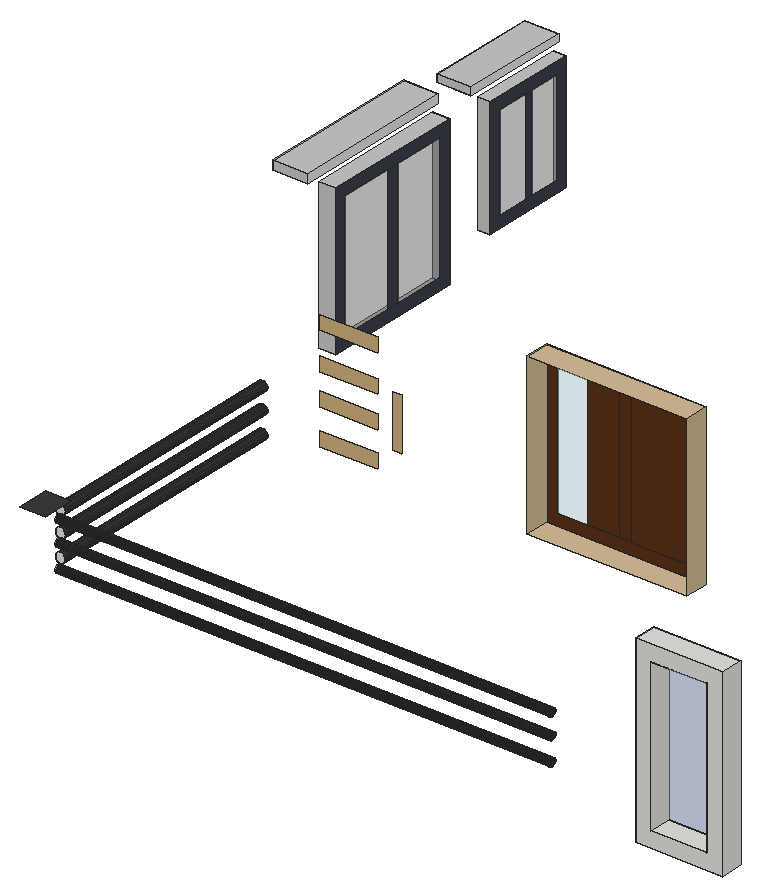
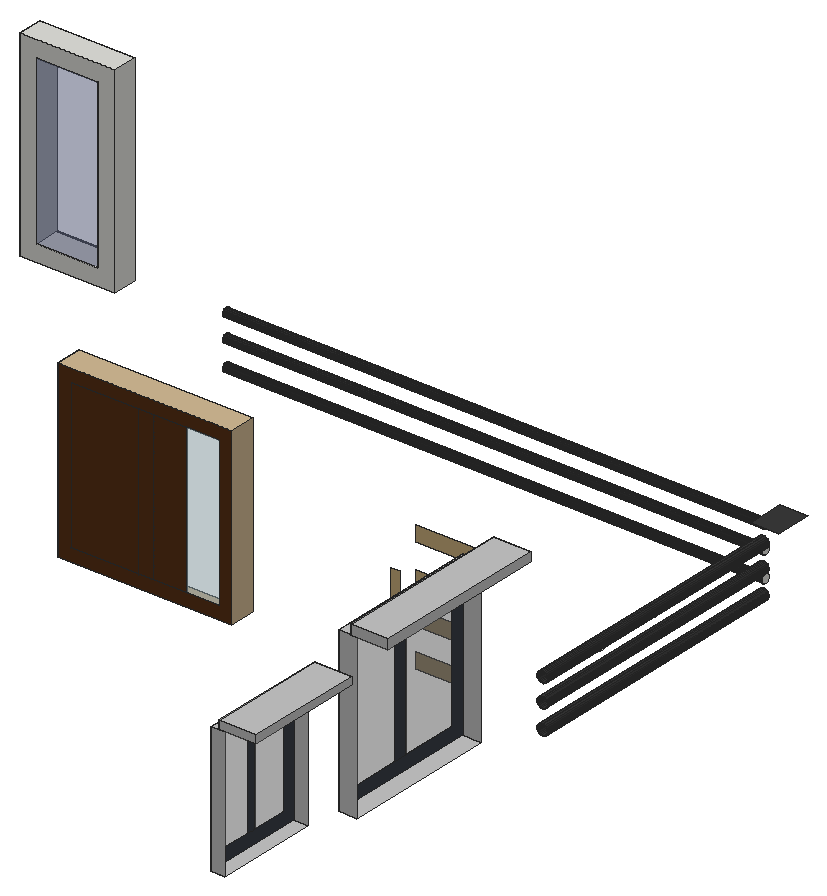
# SketchUp Ruby script. Lengths in inches.
U = 1.inch
M = Sketchup.active_model
def pt(a) = Geom::Point3d.new(a.map { |v| v * U })
def face(e, loops, mat)
  f = e.add_face(loops[0].map { |a| pt(a) })
  loops[1..].each { |l| e.add_face(l.map { |a| pt(a) }).erase! }
  f.material = f.back_material = mat if mat
  f
end
# faces: each face lists its corners as indices into pts; further lists are holes
def faces(e, pts, list, mat = nil) = list.each { |f| face(e, (f[0].is_a?(Array) ? f : [f]).map { |l| l.map { |i| pts[i] } }, mat) }
# xy, xz, yz: faces in a plane at the given z, y or x. An outline is a flat list of corners, or four numbers for a rectangle; further outlines are holes
def ring(l) = l.size == 4 ? [[l[0], l[1]], [l[2], l[1]], [l[2], l[3]], [l[0], l[3]]] : l.each_slice(2).to_a
def flat(e, list, mat, &to3) = list.each { |f| face(e, (f[0].is_a?(Array) ? f : [f]).map { |l| ring(l).map { |u, v| to3.(u, v) } }, mat) }
def xy(e, z, list, mat = nil) = flat(e, list, mat) { |x, y| [x, y, z] }
def xz(e, y, list, mat = nil) = flat(e, list, mat) { |x, z| [x, y, z] }
def yz(e, x, list, mat = nil) = flat(e, list, mat) { |y, z| [x, y, z] }
def lines(e, pts, list) = list.each { |a, b| e.add_line(pt(pts[a]), pt(pts[b])) }
# prism: a flat outline (further loops are holes) pulled along v
def prism(e, loops, v, mat = nil)
  f = face(e, loops, mat); d = Geom::Vector3d.new(v.map { |x| x * U })
  f.pushpull(f.normal.samedirection?(d) ? d.length : -d.length)
end
def box(e, o, s, mat = nil) = prism(e, [[o, [o[0] + s[0], o[1], o[2]], [o[0] + s[0], o[1] + s[1], o[2]], [o[0], o[1] + s[1], o[2]]]], [0, 0, s[2]], mat)
def at(x, y, z, deg = 0) = Geom::Transformation.translation(pt([x, y, z])) * Geom::Transformation.rotation(ORIGIN, Z_AXIS, deg.degrees)
def axes(o, x, y, z) = Geom::Transformation.new([*x, 0, *y, 0, *z, 0, *pt(o).to_a, 1])
def part(name) = M.definitions.add(name)
# library, detail: a bought-in or finely detailed component or shape, given as its bounding box
def library(name, o, s) = part(name).tap { |d| box(d.entities, o, s) }
def detail(e, o, s) = box(e.add_group.entities, o, s)
def put(e, d, t, mat = nil) = e.add_instance(d, t).tap { |i| i.material = mat if mat }
def group(e, t, mat = nil) = e.add_group.tap { |g| g.transformation = t; g.material = mat if mat }.entities
root = M.entities
M.materials.add("[Color M02]").color = [198, 198, 198]
M.materials.add("[Color M07]").color = [58, 58, 58]
M.materials.add("[Formica Beige]").color = [211, 187, 149]
M.materials.add("[Formica Laminate Dark]").color = [59, 63, 71]
M.materials.add("[Translucent Glass Gray]").color = [128, 128, 128]
M.materials["[Translucent Glass Gray]"].alpha = 0.5
M.materials.add("[Translucent Glass Safety]").color = [204, 235, 244]
M.materials["[Translucent Glass Safety]"].alpha = 0.5
M.materials.add("[Translucent Glass Sky Reflection]").color = [126, 138, 183]
M.materials["[Translucent Glass Sky Reflection]"].alpha = 0.52
M.materials.add("[Wood Cherry Original]").color = [89, 50, 24]
M.materials.add("[Wood Floor Light]").color = [204, 176, 127]
xy(root,525.6875,[[382.62,382.59,423.93,393.34]])
xy(root,526.85,[[206.59,538.2,282.28,549.76]],"[Formica Beige]")
xy(root,533.08,[[390.01,382.59,416.53,393.34]])
xy(root,541.0625,[[73.92,580.21,81.98,647.71]],"[Color M02]")
xy(root,544.4375,[[79.76,506.9375,80.23,507,80.66,507.18,81.04,507.47,81.33,507.84,81.51,508.28,81.57,508.75,81.51,509.22,81.33,509.66,81.04,510.03,80.66,510.32,80.23,510.5,79.76,510.5625,79.29,510.5,78.85,510.32,78.48,510.03,78.1875,509.66,78.01,509.22,77.95,508.75,78.01,508.28,78.1875,507.84,78.48,507.47,78.85,507.18,79.29,507]])
xy(root,544.75,[[79.76,478.5,80.23,478.5625,80.66,478.74,81.04,479.03,81.33,479.41,81.51,479.84,81.57,480.3125,81.51,480.78,81.33,481.22,81.04,481.6,80.66,481.88,80.23,482.0625,79.76,482.125,79.29,482.0625,78.85,481.88,78.48,481.6,78.1875,481.22,78.01,480.78,77.95,480.3125,78.01,479.84,78.1875,479.41,78.48,479.03,78.85,478.74,79.29,478.5625]])
xy(root,545.3125,[[79.76,442.375,80.23,442.4375,80.66,442.62,81.04,442.91,81.33,443.28,81.51,443.72,81.57,444.1875,81.51,444.66,81.33,445.09,81.04,445.47,80.66,445.76,80.23,445.9375,79.76,446,79.29,445.9375,78.85,445.76,78.48,445.47,78.1875,445.09,78.01,444.66,77.95,444.1875,78.01,443.72,78.1875,443.28,78.48,442.91,78.85,442.62,79.29,442.4375]])
xy(root,546.625,[[134.48,408.67,134.95,408.73,135.39,408.91,135.76,409.2,136.05,409.58,136.23,410.01,136.29,410.48,136.23,410.95,136.05,411.39,135.76,411.76,135.39,412.05,134.95,412.23,134.48,412.3,134.01,412.23,133.58,412.05,133.2,411.76,132.91,411.39,132.73,410.95,132.67,410.48,132.73,410.01,132.91,409.58,133.2,409.2,133.58,408.91,134.01,408.73]])
xy(root,547.125,[[264.29,408.67,264.76,408.73,265.2,408.91,265.58,409.2,265.86,409.58,266.04,410.01,266.11,410.48,266.04,410.95,265.86,411.39,265.58,411.76,265.2,412.05,264.76,412.23,264.29,412.3,263.82,412.23,263.39,412.05,263.01,411.76,262.72,411.39,262.54,410.95,262.48,410.48,262.54,410.01,262.72,409.58,263.01,409.2,263.39,408.91,263.82,408.73]])
xy(root,547.26,[[199.54,408.67,200.01,408.73,200.45,408.91,200.83,409.2,201.11,409.58,201.29,410.01,201.36,410.48,201.29,410.95,201.11,411.39,200.83,411.76,200.58,411.95,198.51,411.95,198.26,411.76,197.97,411.39,197.79,410.95,197.73,410.48,197.79,410.01,197.97,409.58,198.26,409.2,198.64,408.91,199.07,408.73],[198.51,411.95,200.58,411.95,200.45,412.05,200.01,412.23,199.54,412.3,199.07,412.23,198.64,412.05]])
xy(root,550.0625,[[73.92,674.43,79.92,719.61]],"[Color M02]")
xy(root,551.25,[[73.92,402.63,85.98,418.04]],"[Color M07]")
xy(root,602.54,[[206.59,538.2,282.28,549.76]],"[Formica Beige]")
xy(root,605.29,[[390.01,382.59,416.53,393.34]])
xy(root,606.375,[[73.92,674.43,79.92,719.61]],"[Color M02]")
xy(root,608.8,[[57.67,670.75,73.92,722.6875]],"[Color M02]")
xy(root,611.8125,[[73.92,580.21,81.98,647.71]],"[Color M02]")
xy(root,612.23,[[57.67,670.75,73.92,722.6875]],"[Color M02]")
xy(root,612.6875,[[382.62,382.59,423.93,393.34]])
xy(root,613.9375,[[57.67,573.4375,73.92,651]],"[Color M02]")
xy(root,618.1875,[[57.67,573.4375,73.92,651]],"[Color M02]")
xz(root,382.59,[[[382.62,525.6875,423.93,612.6875],[390.01,533.08,416.53,605.29]]])
xz(root,393.34,[[[382.62,525.6875,423.93,612.6875],[390.01,533.08,416.53,605.29]]])
xz(root,393.34,[[390.01,533.08,416.53,605.29]],"[Translucent Glass Sky Reflection]")
xz(root,418.04,[[80.8,522.8,81.41,522.89,81.99,523.12,82.48,523.5,82.85,523.99,83.09,524.5625,83.17,525.18,83.09,525.79,82.85,526.37,82.48,526.86,81.99,527.24,81.41,527.47,80.8,527.55,80.18,527.47,79.61,527.24,79.12,526.86,78.74,526.37,78.5,525.79,78.42,525.18,78.5,524.5625,78.74,523.99,79.12,523.5,79.61,523.12,80.18,522.89],[80.8,533.37,81.41,533.45,81.99,533.68,82.48,534.0625,82.85,534.55,83.09,535.125,83.17,535.74,83.09,536.36,82.85,536.93,82.48,537.42,81.99,537.8,81.41,538.04,80.8,538.12,80.18,538.04,79.61,537.8,79.12,537.42,78.74,536.93,78.5,536.36,78.42,535.74,78.5,535.125,78.74,534.55,79.12,534.0625,79.61,533.68,80.18,533.45],[80.8,543.3,81.41,543.39,81.99,543.62,82.48,544,82.85,544.49,83.09,545.0625,83.17,545.68,83.09,546.29,82.85,546.87,82.48,547.36,81.99,547.74,81.41,547.97,80.8,548.05,80.18,547.97,79.61,547.74,79.12,547.36,78.74,546.87,78.5,546.29,78.42,545.68,78.5,545.0625,78.74,544.49,79.12,544,79.61,543.62,80.18,543.39]])
xz(root,538.2,[[108.19,529.57,135.69,536.26],[142.77,540.02,146.77,565.12],[108.19,546.38,135.69,553.07],[108.19,561.38,135.69,568.07],[108.19,579.01,135.69,585.69]],"[Wood Floor Light]")
xz(root,549.76,[[212.06,532.3125,226.35,597.07]],"[Translucent Glass Safety]")
xz(root,549.76,[[[206.59,526.85,282.28,602.54],[212.06,532.3125,276.82,597.07]],[226.35,532.3125,240.65,597.07],[240.65,532.3125,246.97,597.07],[246.97,532.3125,276.82,597.07]],"[Wood Cherry Original]")
xz(root,573.4375,[[57.67,613.9375,73.92,618.1875]],"[Color M02]")
xz(root,580.21,[[73.92,541.0625,81.98,611.8125]],"[Color M02]")
xz(root,647.71,[[73.92,541.0625,81.98,611.8125]],"[Color M02]")
xz(root,651,[[57.67,613.9375,73.92,618.1875]],"[Color M02]")
xz(root,670.75,[[57.67,608.8,73.92,612.23]],"[Color M02]")
xz(root,674.43,[[73.92,550.0625,79.92,606.375]],"[Color M02]")
xz(root,719.61,[[73.92,550.0625,79.92,606.375]],"[Color M02]")
xz(root,722.6875,[[57.67,608.8,73.92,612.23]],"[Color M02]")
yz(root,57.67,[[670.75,608.8,722.6875,612.23],[573.4375,613.9375,651,618.1875]],"[Color M02]")
yz(root,73.92,[[670.75,608.8,722.6875,612.23],[573.4375,613.9375,651,618.1875]])
yz(root,79.92,[[[674.43,550.0625,719.61,606.375],[680.02,555.66,714.02,600.78]],[695.45,555.66,699.49,600.78]],"[Formica Laminate Dark]")
yz(root,79.92,[[680.02,555.66,695.45,600.78],[699.49,555.66,714.02,600.78]],"[Translucent Glass Gray]")
yz(root,81.98,[[[580.21,541.0625,647.71,611.8125],[585.81,546.66,642.12,606.22]],[610.89,546.66,616.84,606.22]],"[Formica Laminate Dark]")
yz(root,81.98,[[585.81,546.66,610.89,606.22],[616.84,546.66,642.12,606.22]],"[Translucent Glass Gray]")
yz(root,85.98,[[410.2,524.19,409.75,524.25,409.33,524.43,408.97,524.71,408.6875,525.07,408.51,525.49,408.45,525.94,408.51,526.4,408.6875,526.82,408.97,527.18,409.33,527.46,409.75,527.64,410.2,527.69,410.66,527.64,411.08,527.46,411.44,527.18,411.72,526.82,411.89,526.4,411.95,525.94,411.89,525.49,411.72,525.07,411.44,524.71,411.08,524.43,410.66,524.25],[410.2,535.38,409.75,535.44,409.33,535.62,408.97,535.89,408.6875,536.26,408.51,536.68,408.45,537.13,408.51,537.59,408.6875,538.01,408.97,538.37,409.33,538.65,409.75,538.82,410.2,538.88,410.66,538.82,411.08,538.65,411.44,538.37,411.72,538.01,411.89,537.59,411.95,537.13,411.89,536.68,411.72,536.26,411.44,535.89,411.08,535.62,410.66,535.44],[410.2,545.51,409.75,545.57,409.33,545.74,408.97,546.02,408.6875,546.38,408.51,546.8,408.45,547.26,408.51,547.71,408.6875,548.13,408.97,548.49,409.33,548.77,409.75,548.95,410.2,549.01,410.66,548.95,411.08,548.77,411.44,548.49,411.72,548.13,411.89,547.71,411.95,547.26,411.89,546.8,411.72,546.38,411.44,546.02,411.08,545.74,410.66,545.57]])
yz(root,206.59,[[538.2,526.85,549.76,602.54]],"[Formica Beige]")
yz(root,282.28,[[538.2,526.85,549.76,602.54]],"[Formica Beige]")
yz(root,382.62,[[382.59,525.6875,393.34,612.6875]])
yz(root,390.01,[[382.59,533.08,393.34,605.29]])
yz(root,416.53,[[382.59,533.08,393.34,605.29]])
yz(root,423.93,[[382.59,525.6875,393.34,612.6875]])
p = [[80.8,418.04,522.8],[80.18,418.04,522.89],[80.18,538.2,522.89],[80.8,538.2,522.8],[81.41,418.04,522.89],[81.41,538.2,522.89],
  [79.61,418.04,523.12],[79.61,538.2,523.12],[81.99,418.04,523.12],[81.99,538.2,523.12],[79.12,418.04,523.5],[79.12,538.2,523.5],
  [82.48,418.04,523.5],[82.48,538.2,523.5],[78.74,418.04,523.99],[78.74,538.2,523.99],[82.85,418.04,523.99],[82.85,538.2,523.99],
  [78.5,418.04,524.5625],[78.5,538.2,524.5625],[83.09,418.04,524.5625],[83.09,538.2,524.5625],[85.98,409.75,524.25],[85.98,410.2,524.19],
  [320.99,410.2,524.19],[320.99,409.75,524.25],[85.98,410.66,524.25],[320.99,410.66,524.25],[85.98,409.33,524.43],[320.99,409.33,524.43],
  [85.98,411.08,524.43],[320.99,411.08,524.43],[85.98,408.97,524.71],[320.99,408.97,524.71],[85.98,411.44,524.71],[320.99,411.44,524.71],
  [78.42,418.04,525.18],[78.42,538.2,525.18],[83.17,418.04,525.18],[83.17,538.2,525.18],[85.98,408.6875,525.07],[320.99,408.6875,525.07],
  [85.98,411.72,525.07],[320.99,411.72,525.07],[85.98,408.51,525.49],[320.99,408.51,525.49],[85.98,411.89,525.49],[320.99,411.89,525.49],
  [78.5,418.04,525.79],[78.5,538.2,525.79],[83.09,418.04,525.79],[83.09,538.2,525.79],[85.98,408.45,525.94],[320.99,408.45,525.94],
  [85.98,411.95,525.94],[320.99,411.95,525.94],[78.74,418.04,526.37],[78.74,538.2,526.37],[82.85,418.04,526.37],[82.85,538.2,526.37],
  [85.98,408.51,526.4],[320.99,408.51,526.4],[85.98,411.89,526.4],[320.99,411.89,526.4],[85.98,408.6875,526.82],[320.99,408.6875,526.82],
  [85.98,411.72,526.82],[320.99,411.72,526.82],[79.12,418.04,526.86],[79.12,538.2,526.86],[82.48,418.04,526.86],[82.48,538.2,526.86],
  [85.98,408.97,527.18],[320.99,408.97,527.18],[85.98,411.44,527.18],[320.99,411.44,527.18],[79.61,418.04,527.24],[79.61,538.2,527.24],
  [81.99,418.04,527.24],[81.99,538.2,527.24],[85.98,409.33,527.46],[320.99,409.33,527.46],[85.98,411.08,527.46],[320.99,411.08,527.46],
  [80.18,418.04,527.47],[80.18,538.2,527.47],[81.41,418.04,527.47],[81.41,538.2,527.47],[85.98,409.75,527.64],[320.99,409.75,527.64],
  [85.98,410.66,527.64],[320.99,410.66,527.64],[80.8,418.04,527.55],[80.8,538.2,527.55],[85.98,410.2,527.69],[320.99,410.2,527.69],
  [80.18,418.04,533.45],[79.61,418.04,533.68],[79.61,538.2,533.68],[80.18,538.2,533.45],[80.8,418.04,533.37],[80.8,538.2,533.37],
  [81.41,418.04,533.45],[81.41,538.2,533.45],[81.99,418.04,533.68],[81.99,538.2,533.68],[79.12,418.04,534.0625],[79.12,538.2,534.0625],
  [82.48,418.04,534.0625],[82.48,538.2,534.0625],[78.74,418.04,534.55],[78.74,538.2,534.55],[82.85,418.04,534.55],[82.85,538.2,534.55],
  [78.5,418.04,535.125],[78.5,538.2,535.125],[83.09,418.04,535.125],[83.09,538.2,535.125],[78.42,418.04,535.74],[78.42,538.2,535.74],
  [83.17,418.04,535.74],[83.17,538.2,535.74],[85.98,409.33,535.62],[85.98,409.75,535.44],[320.99,409.75,535.44],[320.99,409.33,535.62],
  [85.98,410.2,535.38],[320.99,410.2,535.38],[85.98,410.66,535.44],[320.99,410.66,535.44],[85.98,411.08,535.62],[320.99,411.08,535.62],
  [85.98,408.97,535.89],[320.99,408.97,535.89],[85.98,411.44,535.89],[320.99,411.44,535.89],[78.5,418.04,536.36],[78.5,538.2,536.36],
  [83.09,418.04,536.36],[83.09,538.2,536.36],[85.98,408.6875,536.26],[320.99,408.6875,536.26],[85.98,411.72,536.26],[320.99,411.72,536.26],
  [85.98,408.51,536.68],[320.99,408.51,536.68],[85.98,411.89,536.68],[320.99,411.89,536.68],[78.74,418.04,536.93],[78.74,538.2,536.93],
  [82.85,418.04,536.93],[82.85,538.2,536.93],[85.98,408.45,537.13],[320.99,408.45,537.13],[85.98,411.95,537.13],[320.99,411.95,537.13],
  [79.12,418.04,537.42],[79.12,538.2,537.42],[82.48,418.04,537.42],[82.48,538.2,537.42],[85.98,408.51,537.59],[320.99,408.51,537.59],
  [85.98,411.89,537.59],[320.99,411.89,537.59],[79.61,418.04,537.8],[79.61,538.2,537.8],[81.99,418.04,537.8],[81.99,538.2,537.8],
  [85.98,408.6875,538.01],[320.99,408.6875,538.01],[85.98,411.72,538.01],[320.99,411.72,538.01],[80.18,418.04,538.04],[80.18,538.2,538.04],
  [81.41,418.04,538.04],[81.41,538.2,538.04],[85.98,408.97,538.37],[320.99,408.97,538.37],[85.98,411.44,538.37],[320.99,411.44,538.37],
  [80.8,418.04,538.12],[80.8,538.2,538.12],[85.98,409.33,538.65],[320.99,409.33,538.65],[85.98,411.08,538.65],[320.99,411.08,538.65],
  [85.98,409.75,538.82],[320.99,409.75,538.82],[85.98,410.66,538.82],[320.99,410.66,538.82],[85.98,410.2,538.88],[320.99,410.2,538.88],
  [80.8,418.04,543.3],[80.18,418.04,543.39],[80.18,538.2,543.39],[80.8,538.2,543.3],[81.41,418.04,543.39],[81.41,538.2,543.39],
  [79.61,418.04,543.62],[79.61,538.2,543.62],[81.99,418.04,543.62],[81.99,538.2,543.62],[79.12,418.04,544],[79.12,538.2,544],
  [82.48,418.04,544],[82.48,538.2,544],[78.74,418.04,544.49],[78.74,538.2,544.49],[82.85,418.04,544.49],[82.85,538.2,544.49],
  [78.5,418.04,545.0625],[78.5,538.2,545.0625],[83.09,418.04,545.0625],[83.09,538.2,545.0625],[78.42,418.04,545.68],[78.42,538.2,545.68],
  [83.17,418.04,545.68],[83.17,538.2,545.68],[85.98,409.75,545.57],[85.98,410.2,545.51],[320.99,410.2,545.51],[320.99,409.75,545.57],
  [85.98,410.66,545.57],[320.99,410.66,545.57],[85.98,409.33,545.74],[320.99,409.33,545.74],[85.98,411.08,545.74],[320.99,411.08,545.74],
  [85.98,408.97,546.02],[320.99,408.97,546.02],[85.98,411.44,546.02],[320.99,411.44,546.02],[78.5,418.04,546.29],[78.5,538.2,546.29],
  [83.09,418.04,546.29],[83.09,538.2,546.29],[85.98,408.6875,546.38],[320.99,408.6875,546.38],[85.98,411.72,546.38],[320.99,411.72,546.38],
  [78.74,418.04,546.87],[78.74,538.2,546.87],[82.85,418.04,546.87],[82.85,538.2,546.87],[85.98,408.51,546.8],[320.99,408.51,546.8],
  [85.98,411.89,546.8],[320.99,411.89,546.8],[85.98,408.45,547.26],[320.99,408.45,547.26],[85.98,411.95,547.26],[198.51,411.95,547.26],
  [200.58,411.95,547.26],[320.99,411.95,547.26],[79.12,418.04,547.36],[79.12,538.2,547.36],[82.48,418.04,547.36],[82.48,538.2,547.36],
  [85.98,408.51,547.71],[320.99,408.51,547.71],[85.98,411.89,547.71],[320.99,411.89,547.71],[79.61,418.04,547.74],[79.61,538.2,547.74],
  [81.99,418.04,547.74],[81.99,538.2,547.74],[85.98,408.6875,548.13],[320.99,408.6875,548.13],[85.98,411.72,548.13],[320.99,411.72,548.13],
  [80.18,418.04,547.97],[80.18,538.2,547.97],[81.41,418.04,547.97],[81.41,538.2,547.97],[80.8,418.04,548.05],[80.8,538.2,548.05],
  [85.98,408.97,548.49],[320.99,408.97,548.49],[85.98,411.44,548.49],[320.99,411.44,548.49],[85.98,409.33,548.77],[320.99,409.33,548.77],
  [85.98,411.08,548.77],[320.99,411.08,548.77],[85.98,409.75,548.95],[320.99,409.75,548.95],[85.98,410.66,548.95],[320.99,410.66,548.95],
  [85.98,410.2,549.01],[320.99,410.2,549.01]]
faces(root,p,[[0,1,2,3],[4,0,3,5],[1,6,7,2],[8,4,5,9],[6,10,11,7],[12,8,9,13],[10,14,15,11],[16,12,13,17],
  [14,18,19,15],[20,16,17,21],[22,23,24,25],[23,26,27,24],[28,22,25,29],[26,30,31,27],[32,28,29,33],[30,34,35,31],
  [18,36,37,19],[38,20,21,39],[40,32,33,41],[34,42,43,35],[44,40,41,45],[42,46,47,43],[36,48,49,37],[50,38,39,51],
  [52,44,45,53],[46,54,55,47],[48,56,57,49],[58,50,51,59],[60,52,53,61],[54,62,63,55],[64,60,61,65],[62,66,67,63],
  [56,68,69,57],[70,58,59,71],[72,64,65,73],[66,74,75,67],[68,76,77,69],[78,70,71,79],[80,72,73,81],[74,82,83,75],
  [76,84,85,77],[86,78,79,87],[88,80,81,89],[82,90,91,83],[84,92,93,85],[92,86,87,93],[94,88,89,95],[90,94,95,91],
  [96,97,98,99],[100,96,99,101],[102,100,101,103],[104,102,103,105],[97,106,107,98],[108,104,105,109],[106,110,111,107],[112,108,109,113],
  [110,114,115,111],[116,112,113,117],[114,118,119,115],[120,116,117,121],[122,123,124,125],[123,126,127,124],[126,128,129,127],[128,130,131,129],
  [132,122,125,133],[130,134,135,131],[118,136,137,119],[138,120,121,139],[140,132,133,141],[134,142,143,135],[144,140,141,145],[142,146,147,143],
  [136,148,149,137],[150,138,139,151],[152,144,145,153],[146,154,155,147],[148,156,157,149],[158,150,151,159],[160,152,153,161],[154,162,163,155],
  [156,164,165,157],[166,158,159,167],[168,160,161,169],[162,170,171,163],[164,172,173,165],[174,166,167,175],[176,168,169,177],[170,178,179,171],
  [172,180,181,173],[180,174,175,181],[182,176,177,183],[178,184,185,179],[186,182,183,187],[184,188,189,185],[190,186,187,191],[188,190,191,189],
  [192,193,194,195],[196,192,195,197],[193,198,199,194],[200,196,197,201],[198,202,203,199],[204,200,201,205],[202,206,207,203],[208,204,205,209],
  [206,210,211,207],[212,208,209,213],[210,214,215,211],[216,212,213,217],[218,219,220,221],[219,222,223,220],[224,218,221,225],[222,226,227,223],
  [228,224,225,229],[226,230,231,227],[214,232,233,215],[234,216,217,235],[236,228,229,237],[230,238,239,231],[232,240,241,233],[242,234,235,243],
  [244,236,237,245],[238,246,247,239],[248,244,245,249],[246,250,251,252,253,247],[240,254,255,241],[256,242,243,257],[258,248,249,259],[250,260,261,253,252,251],
  [254,262,263,255],[264,256,257,265],[266,258,259,267],[260,268,269,261],[262,270,271,263],[272,264,265,273],[270,274,275,271],[274,272,273,275],
  [276,266,267,277],[268,278,279,269],[280,276,277,281],[278,282,283,279],[284,280,281,285],[282,286,287,283],[288,284,285,289],[286,288,289,287]],"[Color M07]")
